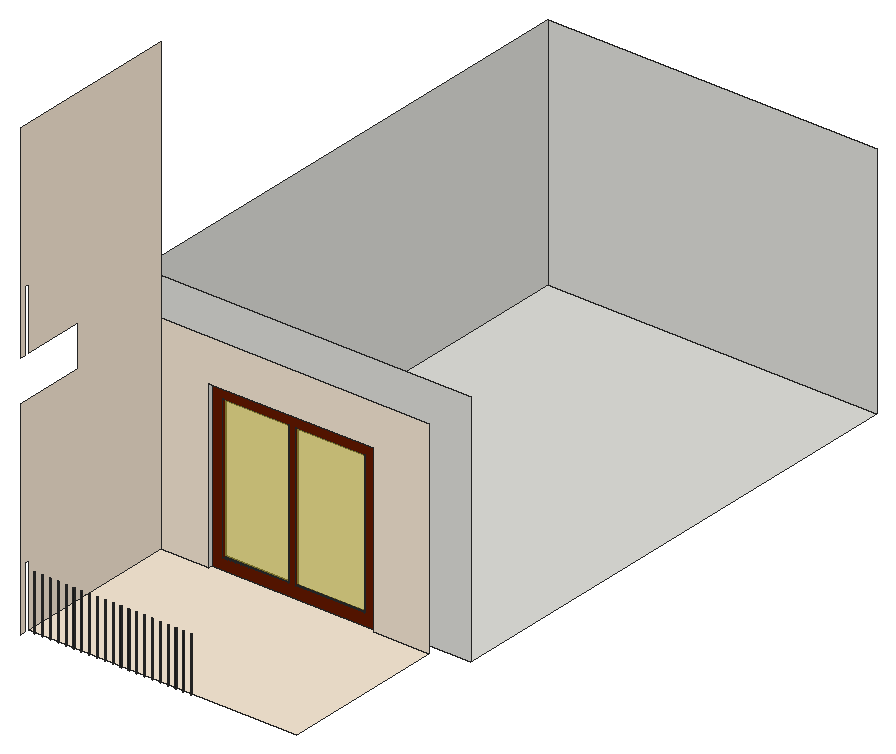
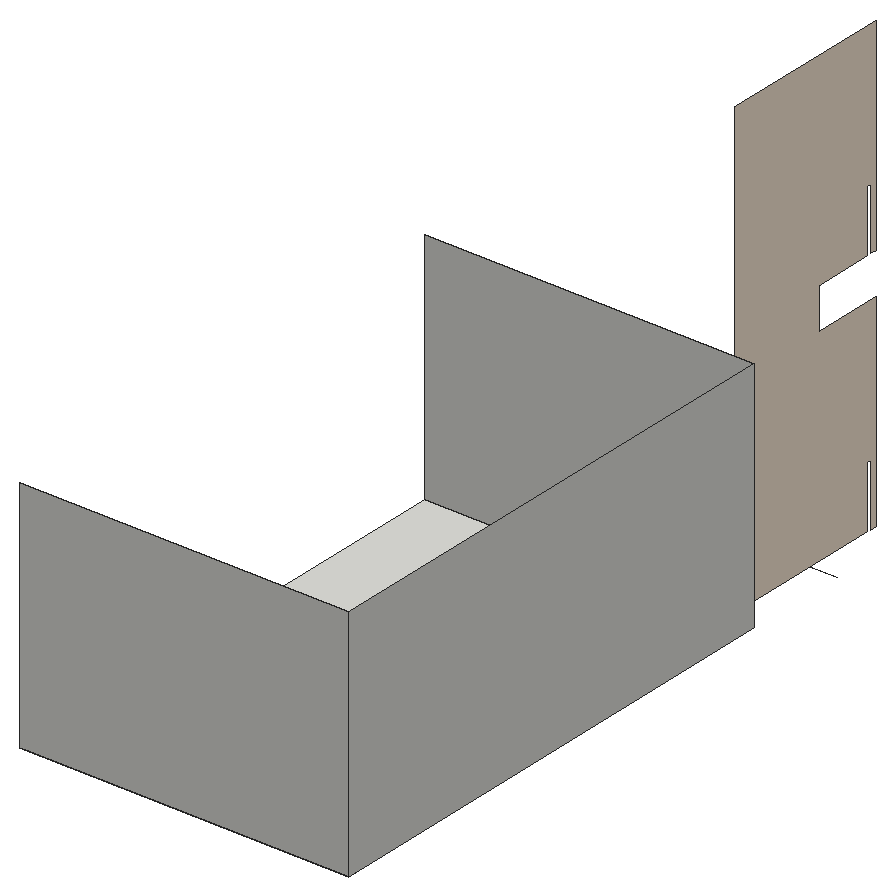
# SketchUp Ruby script. Lengths in inches.
U = 1.inch
M = Sketchup.active_model
def pt(a) = Geom::Point3d.new(a.map { |v| v * U })
def face(e, loops, mat)
  f = e.add_face(loops[0].map { |a| pt(a) })
  loops[1..].each { |l| e.add_face(l.map { |a| pt(a) }).erase! }
  f.material = f.back_material = mat if mat
  f
end
# faces: each face lists its corners as indices into pts; further lists are holes
def faces(e, pts, list, mat = nil) = list.each { |f| face(e, (f[0].is_a?(Array) ? f : [f]).map { |l| l.map { |i| pts[i] } }, mat) }
# xy, xz, yz: faces in a plane at the given z, y or x. An outline is a flat list of corners, or four numbers for a rectangle; further outlines are holes
def ring(l) = l.size == 4 ? [[l[0], l[1]], [l[2], l[1]], [l[2], l[3]], [l[0], l[3]]] : l.each_slice(2).to_a
def flat(e, list, mat, &to3) = list.each { |f| face(e, (f[0].is_a?(Array) ? f : [f]).map { |l| ring(l).map { |u, v| to3.(u, v) } }, mat) }
def xy(e, z, list, mat = nil) = flat(e, list, mat) { |x, y| [x, y, z] }
def xz(e, y, list, mat = nil) = flat(e, list, mat) { |x, z| [x, y, z] }
def yz(e, x, list, mat = nil) = flat(e, list, mat) { |y, z| [x, y, z] }
def lines(e, pts, list) = list.each { |a, b| e.add_line(pt(pts[a]), pt(pts[b])) }
# prism: a flat outline (further loops are holes) pulled along v
def prism(e, loops, v, mat = nil)
  f = face(e, loops, mat); d = Geom::Vector3d.new(v.map { |x| x * U })
  f.pushpull(f.normal.samedirection?(d) ? d.length : -d.length)
end
def box(e, o, s, mat = nil) = prism(e, [[o, [o[0] + s[0], o[1], o[2]], [o[0] + s[0], o[1] + s[1], o[2]], [o[0], o[1] + s[1], o[2]]]], [0, 0, s[2]], mat)
def at(x, y, z, deg = 0) = Geom::Transformation.translation(pt([x, y, z])) * Geom::Transformation.rotation(ORIGIN, Z_AXIS, deg.degrees)
def axes(o, x, y, z) = Geom::Transformation.new([*x, 0, *y, 0, *z, 0, *pt(o).to_a, 1])
def part(name) = M.definitions.add(name)
# library, detail: a bought-in or finely detailed component or shape, given as its bounding box
def library(name, o, s) = part(name).tap { |d| box(d.entities, o, s) }
def detail(e, o, s) = box(e.add_group.entities, o, s)
def put(e, d, t, mat = nil) = e.add_instance(d, t).tap { |i| i.material = mat if mat }
def group(e, t, mat = nil) = e.add_group.tap { |g| g.transformation = t; g.material = mat if mat }.entities
root = M.entities
M.materials.add("[0028_AntiqueWhite]").color = [250, 235, 215]
M.materials.add("[Color B08]").color = [102, 25, 0]
M.materials.add("[Color M08]").color = [30, 30, 30]
M.materials.add("[Translucent Glass Blue]").color = [255, 231, 67]
M.materials["[Translucent Glass Blue]"].alpha = 0.5
c1 = part("Group\#1")
xy(c1.entities,0,[[0,0,71.625,4.3125],[0,4.3125,71.625,7.25]],"[Color B08]")
xy(c1.entities,5.04,[[5.04,0,33.59,4.3125],[36.625,0,66.59,4.3125],[5.04,4.3125,33.59,7.25],[36.625,4.3125,66.59,7.25]],"[Color B08]")
xy(c1.entities,66.59,[[5.04,0,33.59,4.3125],[36.625,0,66.59,4.3125],[5.04,4.3125,33.59,7.25],[36.625,4.3125,66.59,7.25]],"[Color B08]")
xy(c1.entities,71.625,[[0,0,71.625,4.3125],[0,4.3125,71.625,7.25]],"[Color B08]")
xz(c1.entities,0,[[[0,0,71.625,71.625],[36.625,5.04,66.59,66.59],[5.04,5.04,33.59,66.59]]],"[Color B08]")
xz(c1.entities,4.3125,[[[0,0,71.625,71.625],[36.625,5.04,66.59,66.59],[5.04,5.04,33.59,66.59]]],"[Color B08]")
xz(c1.entities,4.3125,[[5.04,5.04,33.59,66.59],[36.625,5.04,66.59,66.59]],"[Translucent Glass Blue]")
xz(c1.entities,7.25,[[[0,0,71.625,71.625],[36.625,5.04,66.59,66.59],[5.04,5.04,33.59,66.59]]],"[Color B08]")
yz(c1.entities,0,[[0,0,4.3125,71.625],[4.3125,0,7.25,71.625]],"[Color B08]")
yz(c1.entities,5.04,[[0,5.04,4.3125,66.59],[4.3125,5.04,7.25,66.59]],"[Color B08]")
yz(c1.entities,33.59,[[0,5.04,4.3125,66.59],[4.3125,5.04,7.25,66.59]],"[Color B08]")
yz(c1.entities,36.625,[[0,5.04,4.3125,66.59],[4.3125,5.04,7.25,66.59]],"[Color B08]")
yz(c1.entities,66.59,[[0,5.04,4.3125,66.59],[4.3125,5.04,7.25,66.59]],"[Color B08]")
yz(c1.entities,71.625,[[0,0,4.3125,71.625],[4.3125,0,7.25,71.625]],"[Color B08]")
xy(root,177,[[35.1875,298.4375,226.3125,592.9375]])
xy(root,177,[[50.75,196.4375,206.5625,196.4375,206.5625,292.44,174.56,292.48,174.5625,296.73,78.6875,296.84,78.68,292.59,50.75,292.625]],"[0028_AntiqueWhite]")
xz(root,195.79,[[54.79,177,54.9375,208.66],[59.35,177,59.5,208.66],[63.92,177,64.0625,208.66],[68.48,177,68.625,208.66],[73.04,177,73.1875,208.66],
  [77.6,177,77.75,208.66],[82.17,177,82.3125,208.66],[86.73,177,86.875,208.66],[91.29,177,91.4375,208.66],[95.85,177,96,208.66],
  [100.42,177,100.5625,208.66],[104.98,177,105.125,208.66],[109.54,177,109.6875,208.66],[114.1,177,114.25,208.66],[118.67,177,118.8125,208.66],
  [123.23,177,123.375,208.66],[127.79,177,127.9375,208.66],[132.35,177,132.5,208.66],[136.92,177,137.0625,208.66],[141.48,177,141.625,208.66],
  [146.04,177,146.1875,208.66]],"[Color M08]")
xz(root,298.4375,[[35.1875,177,226.3125,315]])
xz(root,592.9375,[[35.1875,177,226.3125,315]])
yz(root,35.1875,[[298.4375,177,592.9375,315]])
yz(root,50.75,[[190.5,177,194.125,177,193.58,208.66,193.51,213,196.4375,213,196.4375,177,292.625,177,292.625,441,190.5,441,190.5,321,193.51,321,193.51,357,196.625,357,196.625,321,231.9375,321,231.9375,297,190.5,297]],"[0028_AntiqueWhite]")
p = [[55.31,195.58,177],[55.21,195.68,177],[55.21,195.68,208.66],[55.31,195.58,208.66],[59.87,195.58,177],[59.77,195.68,177],
  [59.77,195.68,208.66],[59.87,195.58,208.66],[64.44,195.58,177],[64.33,195.68,177],[64.33,195.68,208.66],[64.44,195.58,208.66],
  [69,195.58,177],[68.89,195.68,177],[68.89,195.68,208.66],[69,195.58,208.66],[73.56,195.58,177],[73.46,195.68,177],
  [73.46,195.68,208.66],[73.56,195.58,208.66],[78.12,195.58,177],[78.02,195.68,177],[78.02,195.68,208.66],[78.12,195.58,208.66],
  [82.69,195.58,177],[82.58,195.68,177],[82.58,195.68,208.66],[82.69,195.58,208.66],[87.25,195.58,177],[87.14,195.68,177],
  [87.14,195.68,208.66],[87.25,195.58,208.66],[91.81,195.58,177],[91.71,195.68,177],[91.71,195.68,208.66],[91.81,195.58,208.66],
  [96.37,195.58,177],[96.27,195.68,177],[96.27,195.68,208.66],[96.37,195.58,208.66],[100.94,195.58,177],[100.83,195.68,177],
  [100.83,195.68,208.66],[100.94,195.58,208.66],[105.5,195.58,177],[105.39,195.68,177],[105.39,195.68,208.66],[105.5,195.58,208.66],
  [110.06,195.58,177],[109.96,195.68,177],[109.96,195.68,208.66],[110.06,195.58,208.66],[114.62,195.58,177],[114.52,195.68,177],
  [114.52,195.68,208.66],[114.62,195.58,208.66],[119.19,195.58,177],[119.08,195.68,177],[119.08,195.68,208.66],[119.19,195.58,208.66],
  [123.75,195.58,177],[123.64,195.68,177],[123.64,195.68,208.66],[123.75,195.58,208.66],[128.31,195.58,177],[128.21,195.68,177],
  [128.21,195.68,208.66],[128.31,195.58,208.66],[132.87,195.58,177],[132.77,195.68,177],[132.77,195.68,208.66],[132.87,195.58,208.66],
  [137.44,195.58,177],[137.33,195.68,177],[137.33,195.68,208.66],[137.44,195.58,208.66],[142,195.58,177],[141.89,195.68,177],
  [141.89,195.68,208.66],[142,195.58,208.66],[146.56,195.58,177],[146.46,195.68,177],[146.46,195.68,208.66],[146.56,195.58,208.66],
  [54.65,195.75,177],[54.52,195.68,177],[54.52,195.68,208.66],[54.65,195.75,208.66],[55.08,195.75,177],[55.08,195.75,208.66],
  [59.21,195.75,177],[59.08,195.68,177],[59.08,195.68,208.66],[59.21,195.75,208.66],[59.64,195.75,177],[59.64,195.75,208.66],
  [63.77,195.75,177],[63.65,195.68,177],[63.65,195.68,208.66],[63.77,195.75,208.66],[64.2,195.75,177],[64.2,195.75,208.66],
  [68.34,195.75,177],[68.21,195.68,177],[68.21,195.68,208.66],[68.34,195.75,208.66],[68.77,195.75,177],[68.77,195.75,208.66],
  [72.9,195.75,177],[72.77,195.68,177],[72.77,195.68,208.66],[72.9,195.75,208.66],[73.33,195.75,177],[73.33,195.75,208.66],
  [77.46,195.75,177],[77.33,195.68,177],[77.33,195.68,208.66],[77.46,195.75,208.66],[77.89,195.75,177],[77.89,195.75,208.66],
  [82.02,195.75,177],[81.9,195.68,177],[81.9,195.68,208.66],[82.02,195.75,208.66],[82.45,195.75,177],[82.45,195.75,208.66],
  [86.59,195.75,177],[86.46,195.68,177],[86.46,195.68,208.66],[86.59,195.75,208.66],[87.02,195.75,177],[87.02,195.75,208.66],
  [91.15,195.75,177],[91.02,195.68,177],[91.02,195.68,208.66],[91.15,195.75,208.66],[91.58,195.75,177],[91.58,195.75,208.66],
  [95.71,195.75,177],[95.58,195.68,177],[95.58,195.68,208.66],[95.71,195.75,208.66],[96.14,195.75,177],[96.14,195.75,208.66],
  [100.27,195.75,177],[100.15,195.68,177],[100.15,195.68,208.66],[100.27,195.75,208.66],[100.7,195.75,177],[100.7,195.75,208.66],
  [104.84,195.75,177],[104.71,195.68,177],[104.71,195.68,208.66],[104.84,195.75,208.66],[105.27,195.75,177],[105.27,195.75,208.66],
  [109.4,195.75,177],[109.27,195.68,177],[109.27,195.68,208.66],[109.4,195.75,208.66],[109.83,195.75,177],[109.83,195.75,208.66],
  [113.96,195.75,177],[113.83,195.68,177],[113.83,195.68,208.66],[113.96,195.75,208.66],[114.39,195.75,177],[114.39,195.75,208.66],
  [118.52,195.75,177],[118.4,195.68,177],[118.4,195.68,208.66],[118.52,195.75,208.66],[118.95,195.75,177],[118.95,195.75,208.66],
  [123.09,195.75,177],[122.96,195.68,177],[122.96,195.68,208.66],[123.09,195.75,208.66],[123.52,195.75,177],[123.52,195.75,208.66],
  [127.65,195.75,177],[127.52,195.68,177],[127.52,195.68,208.66],[127.65,195.75,208.66],[128.08,195.75,177],[128.08,195.75,208.66],
  [132.21,195.75,177],[132.08,195.68,177],[132.08,195.68,208.66],[132.21,195.75,208.66],[132.64,195.75,177],[132.64,195.75,208.66],
  [136.77,195.75,177],[136.65,195.68,177],[136.65,195.68,208.66],[136.77,195.75,208.66],[137.2,195.75,177],[137.2,195.75,208.66],
  [141.34,195.75,177],[141.21,195.68,177],[141.21,195.68,208.66],[141.34,195.75,208.66],[141.77,195.75,177],[141.77,195.75,208.66],
  [145.9,195.75,177],[145.77,195.68,177],[145.77,195.68,208.66],[145.9,195.75,208.66],[146.33,195.75,177],[146.33,195.75,208.66],
  [54.79,195.79,177],[54.79,195.79,208.66],[54.9375,195.79,177],[54.9375,195.79,208.66],[59.35,195.79,177],[59.35,195.79,208.66],
  [59.5,195.79,177],[59.5,195.79,208.66],[63.92,195.79,177],[63.92,195.79,208.66],[64.0625,195.79,177],[64.0625,195.79,208.66],
  [68.48,195.79,177],[68.48,195.79,208.66],[68.625,195.79,177],[68.625,195.79,208.66],[73.04,195.79,177],[73.04,195.79,208.66],
  [73.1875,195.79,177],[73.1875,195.79,208.66],[77.6,195.79,177],[77.6,195.79,208.66],[77.75,195.79,177],[77.75,195.79,208.66],
  [82.17,195.79,177],[82.17,195.79,208.66],[82.3125,195.79,177],[82.3125,195.79,208.66],[86.73,195.79,177],[86.73,195.79,208.66],
  [86.875,195.79,177],[86.875,195.79,208.66],[91.29,195.79,177],[91.29,195.79,208.66],[91.4375,195.79,177],[91.4375,195.79,208.66],
  [95.85,195.79,177],[95.85,195.79,208.66],[96,195.79,177],[96,195.79,208.66],[100.42,195.79,177],[100.42,195.79,208.66],
  [100.5625,195.79,177],[100.5625,195.79,208.66],[104.98,195.79,177],[104.98,195.79,208.66],[105.125,195.79,177],[105.125,195.79,208.66],
  [109.54,195.79,177],[109.54,195.79,208.66],[109.6875,195.79,177],[109.6875,195.79,208.66],[114.1,195.79,177],[114.1,195.79,208.66],
  [114.25,195.79,177],[114.25,195.79,208.66],[118.67,195.79,177],[118.67,195.79,208.66],[118.8125,195.79,177],[118.8125,195.79,208.66],
  [123.23,195.79,177],[123.23,195.79,208.66],[123.375,195.79,177],[123.375,195.79,208.66],[127.79,195.79,177],[127.79,195.79,208.66],
  [127.9375,195.79,177],[127.9375,195.79,208.66],[132.35,195.79,177],[132.35,195.79,208.66],[132.5,195.79,177],[132.5,195.79,208.66],
  [136.92,195.79,177],[136.92,195.79,208.66],[137.0625,195.79,177],[137.0625,195.79,208.66],[141.48,195.79,177],[141.48,195.79,208.66],
  [141.625,195.79,177],[141.625,195.79,208.66],[146.04,195.79,177],[146.04,195.79,208.66],[146.1875,195.79,177],[146.1875,195.79,208.66],
  [50.75,292.625,177],[78.68,292.59,177],[78.68,292.59,272.875],[174.56,292.48,272.875],[174.56,292.48,177],[206.5625,292.44,177],
  [206.5625,292.44,297],[50.75,292.625,297],[50.75,292.625,296.84],[78.6875,296.84,177],[78.6875,296.84,272.875],[174.5625,296.73,177],
  [174.5625,296.73,272.875],[35.1875,237.9375,177],[50.75,237.9375,177]]
faces(root,p,[[0,1,2,3],[4,5,6,7],[8,9,10,11],[12,13,14,15],[16,17,18,19],[20,21,22,23],[24,25,26,27],[28,29,30,31],
  [32,33,34,35],[36,37,38,39],[40,41,42,43],[44,45,46,47],[48,49,50,51],[52,53,54,55],[56,57,58,59],[60,61,62,63],
  [64,65,66,67],[68,69,70,71],[72,73,74,75],[76,77,78,79],[80,81,82,83],[84,85,86,87],[1,88,89,2],[90,91,92,93],
  [5,94,95,6],[96,97,98,99],[9,100,101,10],[102,103,104,105],[13,106,107,14],[108,109,110,111],[17,112,113,18],[114,115,116,117],
  [21,118,119,22],[120,121,122,123],[25,124,125,26],[126,127,128,129],[29,130,131,30],[132,133,134,135],[33,136,137,34],[138,139,140,141],
  [37,142,143,38],[144,145,146,147],[41,148,149,42],[150,151,152,153],[45,154,155,46],[156,157,158,159],[49,160,161,50],[162,163,164,165],
  [53,166,167,54],[168,169,170,171],[57,172,173,58],[174,175,176,177],[61,178,179,62],[180,181,182,183],[65,184,185,66],[186,187,188,189],
  [69,190,191,70],[192,193,194,195],[73,196,197,74],[198,199,200,201],[77,202,203,78],[204,205,206,207],[81,208,209,82],[210,84,87,211],
  [88,212,213,89],[214,90,93,215],[94,216,217,95],[218,96,99,219],[100,220,221,101],[222,102,105,223],[106,224,225,107],[226,108,111,227],
  [112,228,229,113],[230,114,117,231],[118,232,233,119],[234,120,123,235],[124,236,237,125],[238,126,129,239],[130,240,241,131],[242,132,135,243],
  [136,244,245,137],[246,138,141,247],[142,248,249,143],[250,144,147,251],[148,252,253,149],[254,150,153,255],[154,256,257,155],[258,156,159,259],
  [160,260,261,161],[262,162,165,263],[166,264,265,167],[266,168,171,267],[172,268,269,173],[270,174,177,271],[178,272,273,179],[274,180,183,275],
  [184,276,277,185],[278,186,189,279],[190,280,281,191],[282,192,195,283],[196,284,285,197],[286,198,201,287],[202,288,289,203],[290,204,207,291],
  [208,292,293,209]],"[Color M08]")
faces(root,p,[[294,295,296,297,298,299,300,301,302]],"[0028_AntiqueWhite]")
faces(root,p,[[296,295,303,304],[303,305,306,304]])
lines(root,p,[[307,308]])
put(root,c1,axes([78.68,294.51,177],[1.33857,0,0],[0,0.22,0],[0,0,1.33857]))
